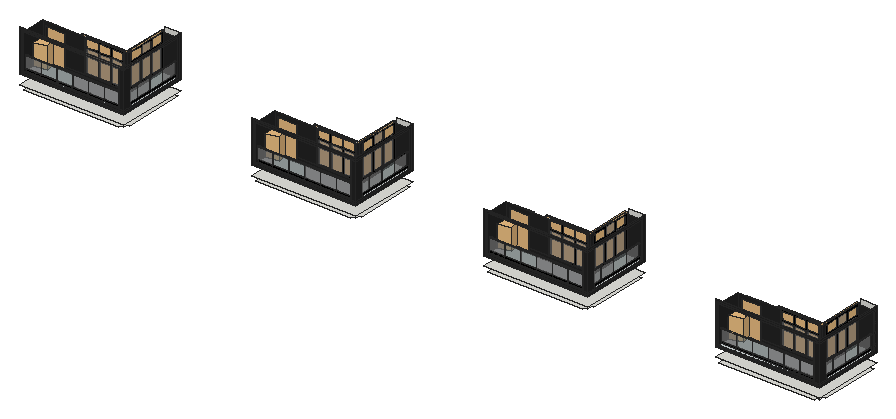
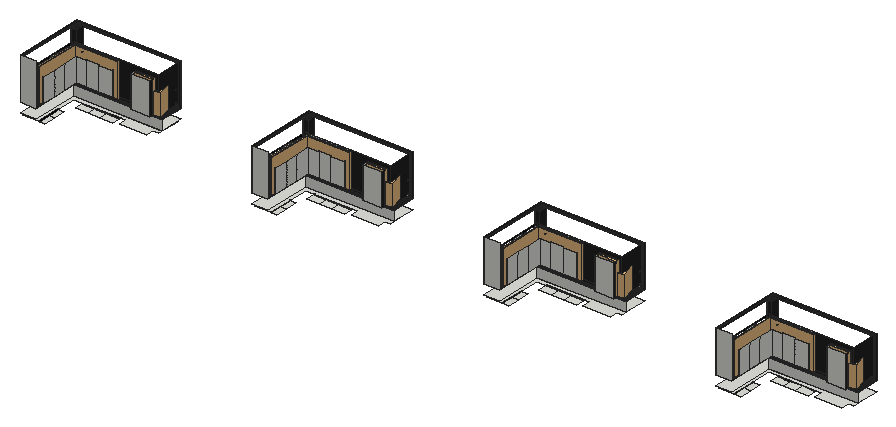
# SketchUp Ruby script. Lengths in inches.
U = 1.inch
M = Sketchup.active_model
def pt(a) = Geom::Point3d.new(a.map { |v| v * U })
def face(e, loops, mat)
  f = e.add_face(loops[0].map { |a| pt(a) })
  loops[1..].each { |l| e.add_face(l.map { |a| pt(a) }).erase! }
  f.material = f.back_material = mat if mat
  f
end
# faces: each face lists its corners as indices into pts; further lists are holes
def faces(e, pts, list, mat = nil) = list.each { |f| face(e, (f[0].is_a?(Array) ? f : [f]).map { |l| l.map { |i| pts[i] } }, mat) }
# xy, xz, yz: faces in a plane at the given z, y or x. An outline is a flat list of corners, or four numbers for a rectangle; further outlines are holes
def ring(l) = l.size == 4 ? [[l[0], l[1]], [l[2], l[1]], [l[2], l[3]], [l[0], l[3]]] : l.each_slice(2).to_a
def flat(e, list, mat, &to3) = list.each { |f| face(e, (f[0].is_a?(Array) ? f : [f]).map { |l| ring(l).map { |u, v| to3.(u, v) } }, mat) }
def xy(e, z, list, mat = nil) = flat(e, list, mat) { |x, y| [x, y, z] }
def xz(e, y, list, mat = nil) = flat(e, list, mat) { |x, z| [x, y, z] }
def yz(e, x, list, mat = nil) = flat(e, list, mat) { |y, z| [x, y, z] }
def lines(e, pts, list) = list.each { |a, b| e.add_line(pt(pts[a]), pt(pts[b])) }
# prism: a flat outline (further loops are holes) pulled along v
def prism(e, loops, v, mat = nil)
  f = face(e, loops, mat); d = Geom::Vector3d.new(v.map { |x| x * U })
  f.pushpull(f.normal.samedirection?(d) ? d.length : -d.length)
end
def box(e, o, s, mat = nil) = prism(e, [[o, [o[0] + s[0], o[1], o[2]], [o[0] + s[0], o[1] + s[1], o[2]], [o[0], o[1] + s[1], o[2]]]], [0, 0, s[2]], mat)
def at(x, y, z, deg = 0) = Geom::Transformation.translation(pt([x, y, z])) * Geom::Transformation.rotation(ORIGIN, Z_AXIS, deg.degrees)
def axes(o, x, y, z) = Geom::Transformation.new([*x, 0, *y, 0, *z, 0, *pt(o).to_a, 1])
def part(name) = M.definitions.add(name)
# library, detail: a bought-in or finely detailed component or shape, given as its bounding box
def library(name, o, s) = part(name).tap { |d| box(d.entities, o, s) }
def detail(e, o, s) = box(e.add_group.entities, o, s)
def put(e, d, t, mat = nil) = e.add_instance(d, t).tap { |i| i.material = mat if mat }
def group(e, t, mat = nil) = e.add_group.tap { |g| g.transformation = t; g.material = mat if mat }.entities
root = M.entities
M.materials.add("Glass Railing Color").color = [198, 198, 198]
M.materials.add("Polycor-Pavers-GEORGIA-MARBLEtm-PEARL-GREY-Tranche-1-4K").color = [207, 214, 215]
M.materials.add("Railing Glass").color = [63, 150, 137]
M.materials["Railing Glass"].alpha = 0.13
M.materials.add("[0136_Charcoal]").color = [35, 35, 35]
M.materials.add("[Color M09]").color = [0, 0, 0]
M.materials.add("[Translucent Glass Gray]").color = [128, 128, 128]
M.materials["[Translucent Glass Gray]"].alpha = 0.5
c1 = library("door by lz",[5.91,-4.92,0],[35.43,6.61,78.74])
c2 = part("Glass Rail Spacer")
box(c2.entities,[-0.5,-0.25,0],[1,0.5,1],"Glass Railing Color")
c3 = part("Group67\#1")
prism(c3.entities,[[[0.54,0,1.27],[0.38,0,1.39],[0.21,0,1.47],[0.01,0,1.5],[-0.18,0,1.48],[-0.37,0,1.41],[-0.52,0,1.29],[-0.64,0,1.13],[-0.72,0,0.96],[-0.75,0,0.76],[-0.73,0,0.57],[-0.66,0,0.38],[-0.54,0,0.23],[-0.38,0,0.11],[-0.21,0,0.03],[-0.01,0,0],[0.18,0,0.02],[0.37,0,0.09],[0.52,0,0.21],[0.64,0,0.37],[0.72,0,0.54],[0.75,0,0.74],[0.73,0,0.93],[0.66,0,1.12]]],[0,242.43,0],"[Color M09]")
c4 = part("Group70\#1")
xy(c4.entities,0,[[-0.5,0,0.5,242.43]],"Glass Railing Color")
xy(c4.entities,4,[[-0.25,0,0.25,242.43]],"Glass Railing Color")
xy(c4.entities,5,[[-0.5,0,-0.25,242.43],[0.25,0,0.5,242.43]],"[Color M09]")
xz(c4.entities,0,[[-0.5,0,0.5,0,0.5,5,0.25,5,0.25,4,-0.25,4,-0.25,5,-0.5,5]],"Glass Railing Color")
xz(c4.entities,242.43,[[-0.5,0,-0.5,5,-0.25,5,-0.25,4,0.25,4,0.25,5,0.5,5,0.5,0]],"Glass Railing Color")
yz(c4.entities,-0.5,[[0,0,242.43,5]],"[Color M09]")
yz(c4.entities,-0.25,[[0,4,242.43,5]],"Glass Railing Color")
yz(c4.entities,0.25,[[0,4,242.43,5]],"[Color M09]")
yz(c4.entities,0.5,[[0,0,242.43,5]],"[Color M09]")
c5 = part("Group71\#1")
box(c5.entities,[-0.1875,0,0],[0.375,39.24,30],"[Translucent Glass Gray]")
c6 = part("Group72\#1")
xy(c6.entities,0,[[-0.1875,0,0.1875,39.24]],"Railing Glass")
xy(c6.entities,30,[[-0.1875,0,0.1875,39.24]],"Railing Glass")
xz(c6.entities,0,[[-0.1875,0,0.1875,30]],"Railing Glass")
xz(c6.entities,39.24,[[-0.1875,0,0.1875,30]],"Railing Glass")
yz(c6.entities,-0.1875,[[0,0,39.24,30]],"Railing Glass")
yz(c6.entities,0.1875,[[0,0,39.24,30]],"[Translucent Glass Gray]")
c7 = part("Group73\#1")
xy(c7.entities,0,[[-0.1875,0,0.1875,39.24]],"Railing Glass")
xy(c7.entities,30,[[-0.1875,0,0.1875,39.24]],"Railing Glass")
xz(c7.entities,0,[[-0.1875,0,0.1875,30]],"Railing Glass")
xz(c7.entities,39.24,[[-0.1875,0,0.1875,30]],"Railing Glass")
yz(c7.entities,-0.1875,[[0,0,39.24,30]],"Railing Glass")
yz(c7.entities,0.1875,[[0,0,39.24,30]],"[Translucent Glass Gray]")
c8 = part("Group74\#1")
box(c8.entities,[-0.1875,0,0],[0.375,39.24,30],"[Translucent Glass Gray]")
c9 = part("Group75\#1")
box(c9.entities,[-0.1875,0,0],[0.375,39.24,30],"[Translucent Glass Gray]")
c10 = part("Group76\#1")
box(c10.entities,[-0.1875,0,0],[0.375,39.24,30],"[Translucent Glass Gray]")
c11 = part("Glass Railing")
put(c11.entities,c2,at(0,0,4))
put(c11.entities,c2,at(40.24,0,4))
put(c11.entities,c2,at(80.48,0,4))
put(c11.entities,c2,at(120.71,0,4))
put(c11.entities,c2,at(160.95,0,4))
put(c11.entities,c2,at(201.19,0,4))
put(c11.entities,c2,at(241.43,0,4))
put(c11.entities,c3,at(-0.5,0,34,-90),"Glass Railing Color")
put(c11.entities,c4,at(-0.5,0,0,-90),"Glass Railing Color")
put(c11.entities,c5,at(0.5,0,4,-90),"Railing Glass")
put(c11.entities,c6,at(40.74,0,4,-90),"Railing Glass")
put(c11.entities,c7,at(80.98,0,4,-90),"Railing Glass")
put(c11.entities,c8,at(121.21,0,4,-90),"Railing Glass")
put(c11.entities,c9,at(161.45,0,4,-90),"Railing Glass")
put(c11.entities,c10,at(201.69,0,4,-90),"Railing Glass")
c12 = part("Group76\#2")
prism(c12.entities,[[[0.54,0,1.27],[0.38,0,1.39],[0.21,0,1.47],[0.01,0,1.5],[-0.18,0,1.48],[-0.37,0,1.41],[-0.52,0,1.29],[-0.64,0,1.13],[-0.72,0,0.96],[-0.75,0,0.76],[-0.73,0,0.57],[-0.66,0,0.38],[-0.54,0,0.23],[-0.38,0,0.11],[-0.21,0,0.03],[-0.01,0,0],[0.18,0,0.02],[0.37,0,0.09],[0.52,0,0.21],[0.64,0,0.37],[0.72,0,0.54],[0.75,0,0.74],[0.73,0,0.93],[0.66,0,1.12]]],[0,161.62,0],"[Color M09]")
c13 = part("Group79\#1")
prism(c13.entities,[[[0.25,0,5],[0.25,0,4],[-0.25,0,4],[-0.25,0,5],[-0.5,0,5],[-0.5,0,0],[0.5,0,0],[0.5,0,5]]],[0,161.62,0],"[Color M09]")
c14 = part("Group80\#1")
box(c14.entities,[-0.1875,0,0],[0.375,39.15,30],"[Translucent Glass Gray]")
c15 = part("Group81\#1")
box(c15.entities,[-0.1875,0,0],[0.375,39.15,30],"[Translucent Glass Gray]")
c16 = part("Group82\#1")
xy(c16.entities,0,[[-0.1875,0,0.1875,39.15]],"Railing Glass")
xy(c16.entities,30,[[-0.1875,0,0.1875,39.15]],"Railing Glass")
xz(c16.entities,0,[[-0.1875,0,0.1875,30]],"Railing Glass")
xz(c16.entities,39.15,[[-0.1875,0,0.1875,30]],"Railing Glass")
yz(c16.entities,-0.1875,[[0,0,39.15,30]],"Railing Glass")
yz(c16.entities,0.1875,[[0,0,39.15,30]],"[Translucent Glass Gray]")
c17 = part("Group83\#1")
box(c17.entities,[-0.1875,0,0],[0.375,39.15,30],"[Translucent Glass Gray]")
c18 = part("Glass Railing\#1")
put(c18.entities,c2,at(0,0,4,90))
put(c18.entities,c2,at(0,40.15,4,90))
put(c18.entities,c2,at(0,80.31,4,90))
put(c18.entities,c2,at(0,120.46,4,90))
put(c18.entities,c2,at(0,160.62,4,90))
put(c18.entities,c12,at(0,-0.5,34),"Glass Railing Color")
put(c18.entities,c13,at(0,-0.5,0),"[Color M09]")
put(c18.entities,c14,at(0,0.5,4),"Railing Glass")
put(c18.entities,c15,at(0,40.65,4),"Railing Glass")
put(c18.entities,c16,at(0,80.81,4),"Railing Glass")
put(c18.entities,c17,at(0,120.96,4),"Railing Glass")
c19 = library("cay+chuoi",[36.12,19.66,0.52],[32.73,35.6,54.38])
c20 = library("curtain",[-132.09,64.9,20.5],[94.35,4.27,84.68])
xy(root,118.1875,[[501.6,560.12,516.04,589.16],[1091.41,560.12,1105.85,589.16],[1681.23,560.12,1695.66,589.16],[2271.04,560.12,2285.48,589.16],[501.6,589.16,516.04,620.2],
  [1091.41,589.16,1105.85,620.2],[1681.23,589.16,1695.66,620.2],[2271.04,589.16,2285.48,620.2]])
xy(root,118.87,[[302.04,449.7,302.04,509.7,315.54,509.7,315.54,530.01,384.73,530.01,384.73,509.7,518.04,509.7,518.04,620.88,557.59,620.88,557.59,468.65,551.21,468.65,551.21,457.2,544.21,457.2,544.21,449.7],[891.85,449.7,891.85,509.7,905.35,509.7,905.35,530.01,974.54,530.01,974.54,509.7,1107.85,509.7,1107.85,620.88,1147.4,620.88,1147.4,468.65,1141.02,468.65,1141.02,457.2,1134.02,457.2,1134.02,449.7],[1481.66,449.7,1481.66,509.7,1495.16,509.7,1495.16,530.01,1564.35,530.01,1564.35,509.7,1697.66,509.7,1697.66,620.88,1737.22,620.88,1737.22,468.65,1730.83,468.65,1730.83,457.2,1723.83,457.2,1723.83,449.7],[2071.48,449.7,2071.48,509.7,2084.98,509.7,2084.98,530.01,2154.16,530.01,2154.16,509.7,2287.48,509.7,2287.48,620.88,2327.03,620.88,2327.03,468.65,2320.65,468.65,2320.65,457.2,2313.65,457.2,2313.65,449.7],[398.04,512.7,430.93,533.7],
  [430.93,512.7,461.15,533.7],[461.15,512.7,494.04,533.7],[987.85,512.7,1020.74,533.7],[1020.74,512.7,1050.96,533.7],[1050.96,512.7,1083.85,533.7],
  [1577.66,512.7,1610.56,533.7],[1610.56,512.7,1640.77,533.7],[1640.77,512.7,1673.66,533.7],[2167.48,512.7,2200.37,533.7],[2200.37,512.7,2230.58,533.7],
  [2230.58,512.7,2263.48,533.7]])
xy(root,118.87,[[398.04,509.7,494.04,512.7],[987.85,509.7,1083.85,512.7],[1577.66,509.7,1673.66,512.7],[2167.48,509.7,2263.48,512.7],[516.04,559.44,518.04,620.88],
  [1105.85,559.44,1107.85,620.88],[1695.66,559.44,1697.66,620.88],[2285.48,559.44,2287.48,620.88]],"[Color M09]")
xy(root,127.6875,[[293.22,449.7,557.59,449.7,557.59,629.7,518.04,629.7,518.04,509.7,293.22,509.7],[883.03,449.7,1147.4,449.7,1147.4,629.7,1107.85,629.7,1107.85,509.7,883.03,509.7],[1472.84,449.7,1737.22,449.7,1737.22,629.7,1697.66,629.7,1697.66,509.7,1472.84,509.7],[2062.65,449.7,2327.03,449.7,2327.03,629.7,2287.48,629.7,2287.48,509.7,2062.65,509.7]])
xy(root,151.6875,[[293.22,449.7,557.59,509.7],[883.03,449.7,1147.4,509.7],[1472.84,449.7,1737.22,509.7],[2062.65,449.7,2327.03,509.7],[518.04,509.7,557.59,629.7],
  [1107.85,509.7,1147.4,629.7],[1697.66,509.7,1737.22,629.7],[2287.48,509.7,2327.03,629.7]],"[0136_Charcoal]")
xy(root,155.16,[[296.69,449.7,557.59,450.7],[886.5,449.7,1147.4,450.7],[1476.32,449.7,1737.22,450.7],[2066.13,449.7,2327.03,450.7],[556.59,450.7,557.59,625.64],
  [1146.4,450.7,1147.4,625.64],[1736.22,450.7,1737.22,625.64],[2326.03,450.7,2327.03,625.64]],"[0136_Charcoal]")
xy(root,156.3,[[297.83,449.7,557.59,450.7],[887.64,449.7,1147.4,450.7],[1477.46,449.7,1737.22,450.7],[2067.27,449.7,2327.03,450.7]],"[0136_Charcoal]")
xy(root,159.6875,[[311.04,509.7,359.04,525.45],[900.85,509.7,948.85,525.45],[1490.66,509.7,1538.66,525.45],[2080.48,509.7,2128.48,525.45]])
xy(root,159.6875,[[302.04,449.7,557.59,449.7,557.59,621.7,518.04,621.7,518.04,509.7,302.04,509.7],[891.85,449.7,1147.4,449.7,1147.4,621.7,1107.85,621.7,1107.85,509.7,891.85,509.7],[1481.66,449.7,1737.22,449.7,1737.22,621.7,1697.66,621.7,1697.66,509.7,1481.66,509.7],[2071.48,449.7,2327.03,449.7,2327.03,621.7,2287.48,621.7,2287.48,509.7,2071.48,509.7]],"Polycor-Pavers-GEORGIA-MARBLEtm-PEARL-GREY-Tranche-1-4K")
xy(root,165.6875,[[410.04,509.7,509.04,511.7],[999.85,509.7,1098.85,511.7],[1589.66,509.7,1688.66,511.7],[2179.48,509.7,2278.48,511.7],[503.73,519.34,515.04,555.96],
  [515.04,519.34,518.04,621.7],[1093.54,519.34,1104.85,555.96],[1104.85,519.34,1107.85,621.7],[1683.35,519.34,1694.66,555.96],[1694.66,519.34,1697.66,621.7],
  [2273.16,519.34,2284.48,555.96],[2284.48,519.34,2287.48,621.7],[503.73,555.96,515.04,588.08],[1093.54,555.96,1104.85,588.08],[1683.35,555.96,1694.66,588.08],
  [2273.16,555.96,2284.48,588.08],[503.73,588.08,515.04,621.7],[1093.54,588.08,1104.85,621.7],[1683.35,588.08,1694.66,621.7],[2273.16,588.08,2284.48,621.7]])
xy(root,166.1875,[[410.54,511.7,445.2,519.01],[445.2,511.7,476.87,519.01],[476.87,511.7,508.54,519.01],[1000.35,511.7,1035.02,519.01],[1035.02,511.7,1066.68,519.01],
  [1066.68,511.7,1098.35,519.01],[1590.16,511.7,1624.83,519.01],[1624.83,511.7,1656.5,519.01],[1656.5,511.7,1688.16,519.01],[2179.98,511.7,2214.64,519.01],
  [2214.64,511.7,2246.31,519.01],[2246.31,511.7,2277.98,519.01]])
xy(root,167.6875,[[445.2,509.7,475.37,511.7],[476.87,509.7,507.04,511.7],[1035.02,509.7,1065.18,511.7],[1066.68,509.7,1096.85,511.7],[1624.83,509.7,1655,511.7],
  [1656.5,509.7,1686.66,511.7],[2214.64,509.7,2244.81,511.7],[2246.31,509.7,2276.48,511.7]])
xy(root,167.6875,[[412.04,509.7,443.7,511.7],[1001.85,509.7,1033.52,511.7],[1591.66,509.7,1623.33,511.7],[2181.48,509.7,2213.14,511.7],[515.04,521.34,518.04,553.96],
  [1104.85,521.34,1107.85,553.96],[1694.66,521.34,1697.66,553.96],[2284.48,521.34,2287.48,553.96],[515.04,555.96,518.04,586.08],[1104.85,555.96,1107.85,586.08],
  [1694.66,555.96,1697.66,586.08],[2284.48,555.96,2287.48,586.08],[515.04,588.08,518.04,619.7],[1104.85,588.08,1107.85,619.7],[1694.66,588.08,1697.66,619.7],
  [2284.48,588.08,2287.48,619.7]],"[Color M09]")
xz(root,449.7,[[293.22,151.6875,557.59,151.6875,557.59,155.16,296.69,155.16,296.69,256.21,557.59,256.21,557.59,259.6875,293.22,259.6875],[883.03,151.6875,1147.4,151.6875,1147.4,155.16,886.5,155.16,886.5,256.21,1147.4,256.21,1147.4,259.6875,883.03,259.6875],[1472.84,151.6875,1737.22,151.6875,1737.22,155.16,1476.32,155.16,1476.32,256.21,1737.22,256.21,1737.22,259.6875,1472.84,259.6875],[2062.65,151.6875,2327.03,151.6875,2327.03,155.16,2066.13,155.16,2066.13,256.21,2327.03,256.21,2327.03,259.6875,2062.65,259.6875],[297.83,156.3,557.59,156.3,557.59,159.6875,302.04,159.6875,302.04,251.6875,557.59,251.6875,557.59,255.07,297.83,255.07],
  [887.64,156.3,1147.4,156.3,1147.4,159.6875,891.85,159.6875,891.85,251.6875,1147.4,251.6875,1147.4,255.07,887.64,255.07],[1477.46,156.3,1737.22,156.3,1737.22,159.6875,1481.66,159.6875,1481.66,251.6875,1737.22,251.6875,1737.22,255.07,1477.46,255.07],[2067.27,156.3,2327.03,156.3,2327.03,159.6875,2071.48,159.6875,2071.48,251.6875,2327.03,251.6875,2327.03,255.07,2067.27,255.07]],"[0136_Charcoal]")
xz(root,450.7,[[296.69,155.16,556.59,155.16,556.59,156.3,297.83,156.3,297.83,255.07,556.59,255.07,556.59,256.21,296.69,256.21],[886.5,155.16,1146.4,155.16,1146.4,156.3,887.64,156.3,887.64,255.07,1146.4,255.07,1146.4,256.21,886.5,256.21],[1476.32,155.16,1736.22,155.16,1736.22,156.3,1477.46,156.3,1477.46,255.07,1736.22,255.07,1736.22,256.21,1476.32,256.21],[2066.13,155.16,2326.03,155.16,2326.03,156.3,2067.27,156.3,2067.27,255.07,2326.03,255.07,2326.03,256.21,2066.13,256.21]],"[0136_Charcoal]")
xz(root,509.7,[[293.22,127.6875,518.04,151.6875],[883.03,127.6875,1107.85,151.6875],[1472.84,127.6875,1697.66,151.6875],[2062.65,127.6875,2287.48,151.6875],[302.04,159.6875,311.04,165.6875],
  [891.85,159.6875,900.85,165.6875],[1481.66,159.6875,1490.66,165.6875],[2071.48,159.6875,2080.48,165.6875]])
xz(root,509.7,[[359.04,159.6875,518.04,165.6875],[948.85,159.6875,1107.85,165.6875],[1538.66,159.6875,1697.66,165.6875],[2128.48,159.6875,2287.48,165.6875],[302.04,165.6875,311.04,165.6875,311.04,240.6,359.04,240.6,359.04,165.6875,410.04,165.6875,410.04,251.6875,302.04,251.6875],
  [509.04,165.6875,518.04,251.6875],[891.85,165.6875,900.85,165.6875,900.85,240.6,948.85,240.6,948.85,165.6875,999.85,165.6875,999.85,251.6875,891.85,251.6875],[1098.85,165.6875,1107.85,251.6875],[1481.66,165.6875,1490.66,165.6875,1490.66,240.6,1538.66,240.6,1538.66,165.6875,1589.66,165.6875,1589.66,251.6875,1481.66,251.6875],[1688.66,165.6875,1697.66,251.6875],
  [2071.48,165.6875,2080.48,165.6875,2080.48,240.6,2128.48,240.6,2128.48,165.6875,2179.48,165.6875,2179.48,251.6875,2071.48,251.6875],[2278.48,165.6875,2287.48,251.6875]],"[0136_Charcoal]")
xz(root,509.7,[[[410.04,165.6875,509.04,251.6875],[412.04,227.74,412.04,249.6875,507.04,249.6875,507.04,227.74,476.87,227.74,476.87,249.6875,475.37,249.6875,475.37,227.74,445.2,227.74,445.2,249.6875,443.7,249.6875,443.7,227.74],[412.04,167.6875,443.7,225.74],[476.87,167.6875,507.04,225.74],[445.2,167.6875,475.37,225.74]],[[999.85,165.6875,1098.85,251.6875],[1001.85,227.74,1001.85,249.6875,1096.85,249.6875,1096.85,227.74,1066.68,227.74,1066.68,249.6875,1065.18,249.6875,1065.18,227.74,1035.02,227.74,1035.02,249.6875,1033.52,249.6875,1033.52,227.74],[1001.85,167.6875,1033.52,225.74],[1066.68,167.6875,1096.85,225.74],[1035.02,167.6875,1065.18,225.74]],[[1589.66,165.6875,1688.66,251.6875],[1591.66,227.74,1591.66,249.6875,1686.66,249.6875,1686.66,227.74,1656.5,227.74,1656.5,249.6875,1655,249.6875,1655,227.74,1624.83,227.74,1624.83,249.6875,1623.33,249.6875,1623.33,227.74],[1591.66,167.6875,1623.33,225.74],[1656.5,167.6875,1686.66,225.74],[1624.83,167.6875,1655,225.74]],[[2179.48,165.6875,2278.48,251.6875],[2181.48,227.74,2181.48,249.6875,2276.48,249.6875,2276.48,227.74,2246.31,227.74,2246.31,249.6875,2244.81,249.6875,2244.81,227.74,2214.64,227.74,2214.64,249.6875,2213.14,249.6875,2213.14,227.74],[2181.48,167.6875,2213.14,225.74],[2246.31,167.6875,2276.48,225.74],[2214.64,167.6875,2244.81,225.74]]],"[Color M09]")
xz(root,510.7,[[476.87,165.6875,509.04,225.74],[1066.68,165.6875,1098.85,225.74],[1656.5,165.6875,1688.66,225.74],[2246.31,165.6875,2278.48,225.74],[412.04,167.6875,443.7,225.74],
  [445.2,167.6875,475.37,225.74],[1001.85,167.6875,1033.52,225.74],[1035.02,167.6875,1065.18,225.74],[1591.66,167.6875,1623.33,225.74],[1624.83,167.6875,1655,225.74],
  [2181.48,167.6875,2213.14,225.74],[2214.64,167.6875,2244.81,225.74]],"[Translucent Glass Gray]")
xz(root,511.7,[[[410.04,165.6875,509.04,251.6875],[410.54,166.1875,508.54,249.6875]],[[999.85,165.6875,1098.85,251.6875],[1000.35,166.1875,1098.35,249.6875]],[[1589.66,165.6875,1688.66,251.6875],[1590.16,166.1875,1688.16,249.6875]],[[2179.48,165.6875,2278.48,251.6875],[2179.98,166.1875,2277.98,249.6875]],[410.54,166.1875,412.04,227.74],
  [412.04,166.1875,443.7,167.6875],[443.7,166.1875,445.2,225.74],[445.2,166.1875,475.37,167.6875],[475.37,166.1875,476.87,227.61],[476.87,166.1875,508.54,167.6875],
  [1000.35,166.1875,1001.85,227.74],[1001.85,166.1875,1033.52,167.6875],[1033.52,166.1875,1035.02,225.74],[1035.02,166.1875,1065.18,167.6875],[1065.18,166.1875,1066.68,227.61],
  [1066.68,166.1875,1098.35,167.6875],[1590.16,166.1875,1591.66,227.74],[1591.66,166.1875,1623.33,167.6875],[1623.33,166.1875,1624.83,225.74],[1624.83,166.1875,1655,167.6875],
  [1655,166.1875,1656.5,227.61],[1656.5,166.1875,1688.16,167.6875],[2179.98,166.1875,2181.48,227.74],[2181.48,166.1875,2213.14,167.6875],[2213.14,166.1875,2214.64,225.74],
  [2214.64,166.1875,2244.81,167.6875],[2244.81,166.1875,2246.31,227.61],[2246.31,166.1875,2277.98,167.6875],[507.04,167.6875,508.54,225.74],[1096.85,167.6875,1098.35,225.74],
  [1686.66,167.6875,1688.16,225.74],[2276.48,167.6875,2277.98,225.74]])
xz(root,519.01,[[410.54,166.1875,445.2,225.74],[445.2,166.1875,476.87,227.61],[476.87,166.1875,508.54,225.74],[1000.35,166.1875,1035.02,225.74],[1035.02,166.1875,1066.68,227.61],
  [1066.68,166.1875,1098.35,225.74],[1590.16,166.1875,1624.83,225.74],[1624.83,166.1875,1656.5,227.61],[1656.5,166.1875,1688.16,225.74],[2179.98,166.1875,2214.64,225.74],
  [2214.64,166.1875,2246.31,227.61],[2246.31,166.1875,2277.98,225.74]])
xz(root,519.34,[[503.73,165.6875,515.04,224.74],[515.04,165.6875,518.04,251.6875],[1093.54,165.6875,1104.85,224.74],[1104.85,165.6875,1107.85,251.6875],[1683.35,165.6875,1694.66,224.74],
  [1694.66,165.6875,1697.66,251.6875],[2273.16,165.6875,2284.48,224.74],[2284.48,165.6875,2287.48,251.6875]])
xz(root,521.34,[[515.04,167.6875,518.04,225.74],[1104.85,167.6875,1107.85,225.74],[1694.66,167.6875,1697.66,225.74],[2284.48,167.6875,2287.48,225.74]],"[Color M09]")
xz(root,525.45,[[311.04,159.6875,359.04,240.6],[900.85,159.6875,948.85,240.6],[1490.66,159.6875,1538.66,240.6],[2080.48,159.6875,2128.48,240.6]])
xz(root,553.96,[[515.04,167.6875,518.04,225.74],[1104.85,167.6875,1107.85,225.74],[1694.66,167.6875,1697.66,225.74],[2284.48,167.6875,2287.48,225.74]],"[Color M09]")
xz(root,555.96,[[515.04,167.6875,518.04,225.74],[1104.85,167.6875,1107.85,225.74],[1694.66,167.6875,1697.66,225.74],[2284.48,167.6875,2287.48,225.74]],"[Color M09]")
xz(root,586.08,[[515.04,167.6875,518.04,225.74],[1104.85,167.6875,1107.85,225.74],[1694.66,167.6875,1697.66,225.74],[2284.48,167.6875,2287.48,225.74]],"[Color M09]")
xz(root,588.08,[[515.04,167.6875,518.04,225.74],[1104.85,167.6875,1107.85,225.74],[1694.66,167.6875,1697.66,225.74],[2284.48,167.6875,2287.48,225.74]],"[Color M09]")
xz(root,619.7,[[515.04,167.6875,518.04,225.74],[1104.85,167.6875,1107.85,225.74],[1694.66,167.6875,1697.66,225.74],[2284.48,167.6875,2287.48,225.74]],"[Color M09]")
xz(root,621.7,[[503.73,165.6875,515.04,224.74],[515.04,165.6875,518.04,251.6875],[1093.54,165.6875,1104.85,224.74],[1104.85,165.6875,1107.85,251.6875],[1683.35,165.6875,1694.66,224.74],
  [1694.66,165.6875,1697.66,251.6875],[2273.16,165.6875,2284.48,224.74],[2284.48,165.6875,2287.48,251.6875]])
xz(root,621.7,[[518.04,159.6875,557.59,251.6875],[1107.85,159.6875,1147.4,251.6875],[1697.66,159.6875,1737.22,251.6875],[2287.48,159.6875,2327.03,251.6875]],"[0136_Charcoal]")
xz(root,624.51,[[556.59,157.14,557.59,255.07],[1146.4,157.14,1147.4,255.07],[1736.22,157.14,1737.22,255.07],[2326.03,157.14,2327.03,255.07]])
xz(root,625.64,[[556.59,155.16,557.59,155.71],[1146.4,155.16,1147.4,155.71],[1736.22,155.16,1737.22,155.71],[2326.03,155.16,2327.03,155.71],[556.59,155.71,557.59,256.21],
  [1146.4,155.71,1147.4,256.21],[1736.22,155.71,1737.22,256.21],[2326.03,155.71,2327.03,256.21]],"[0136_Charcoal]")
xz(root,629.7,[[518.04,151.6875,557.59,259.6875],[1107.85,151.6875,1147.4,259.6875],[1697.66,151.6875,1737.22,259.6875],[2287.48,151.6875,2327.03,259.6875]])
yz(root,296.69,[[449.7,155.16,450.7,256.21]],"[0136_Charcoal]")
yz(root,297.83,[[449.7,156.3,450.7,255.07]],"[0136_Charcoal]")
yz(root,302.04,[[449.7,159.6875,509.7,251.6875]],"[0136_Charcoal]")
yz(root,311.04,[[509.7,159.6875,525.45,240.6]],"[0136_Charcoal]")
yz(root,359.04,[[509.7,159.6875,525.45,240.6]])
yz(root,410.04,[[509.7,165.6875,511.7,251.6875]])
yz(root,410.54,[[511.7,166.1875,519.01,227.74]])
yz(root,412.04,[[509.7,167.6875,511.7,225.74]],"[Color M09]")
yz(root,443.7,[[509.7,167.6875,511.7,225.74]],"[Color M09]")
yz(root,445.2,[[509.7,167.6875,511.7,225.74]],"[Color M09]")
yz(root,475.37,[[509.7,167.6875,511.7,225.74]],"[Color M09]")
yz(root,476.87,[[509.7,167.6875,511.7,225.74]],"[Color M09]")
yz(root,503.73,[[519.34,165.6875,555.96,224.74],[555.96,165.6875,588.08,224.74],[588.08,165.6875,621.7,224.74]])
yz(root,507.04,[[509.7,167.6875,511.7,225.74]],"[Color M09]")
yz(root,508.54,[[511.7,166.1875,519.01,225.74]],"[Color M09]")
yz(root,509.04,[[509.7,165.6875,511.7,251.6875]])
yz(root,515.04,[[519.34,165.6875,519.34,168.6875,521.34,168.6875,521.34,167.6875,552.96,167.6875,552.96,165.6875],[552.96,165.6875,552.96,167.6875,553.96,167.6875,553.96,224.74,555.96,224.74,555.96,165.6875],[555.96,165.6875,585.08,167.6875],[585.08,165.6875,585.08,167.6875,586.08,167.6875,586.08,224.74,588.08,224.74,588.08,165.6875],[588.08,165.6875,618.7,167.6875],
  [618.7,165.6875,618.7,167.6875,619.7,167.6875,619.7,224.74,621.7,224.74,621.7,165.6875]])
yz(root,516.54,[[521.34,167.6875,553.96,225.74],[555.96,167.6875,586.08,225.74],[588.08,167.6875,619.7,225.74],[555.96,225.74,586.08,249.6875]],"[Translucent Glass Gray]")
yz(root,518.04,[[509.7,159.6875,519.34,251.6875],[519.34,159.6875,621.7,165.6875]],"[0136_Charcoal]")
yz(root,518.04,[[[519.34,165.6875,621.7,251.6875],[521.34,167.6875,553.96,225.74],[588.08,167.6875,619.7,225.74],[555.96,167.6875,586.08,225.74],[521.34,227.74,553.96,249.6875],[588.08,227.74,619.7,249.6875],[555.96,227.74,586.08,249.6875]]],"[Color M09]")
yz(root,556.59,[[450.7,155.16,625.64,155.16,625.64,256.21,450.7,256.21,450.7,255.07,624.51,255.07,624.51,157.14,450.7,156.3]],"[0136_Charcoal]")
yz(root,557.59,[[449.7,151.6875,629.7,151.6875,629.7,259.6875,449.7,259.6875,449.7,256.21,625.64,256.21,625.64,155.16,449.7,155.16],[449.7,156.3,450.7,156.3,624.51,157.14,624.51,255.07,449.7,255.07,449.7,251.6875,621.7,251.6875,621.7,159.6875,449.7,159.6875]],"[0136_Charcoal]")
yz(root,886.5,[[449.7,155.16,450.7,256.21]],"[0136_Charcoal]")
yz(root,887.64,[[449.7,156.3,450.7,255.07]],"[0136_Charcoal]")
yz(root,891.85,[[449.7,159.6875,509.7,251.6875]],"[0136_Charcoal]")
yz(root,900.85,[[509.7,159.6875,525.45,240.6]],"[0136_Charcoal]")
yz(root,948.85,[[509.7,159.6875,525.45,240.6]])
yz(root,999.85,[[509.7,165.6875,511.7,251.6875]])
yz(root,1000.35,[[511.7,166.1875,519.01,227.74]])
yz(root,1001.85,[[509.7,167.6875,511.7,225.74]],"[Color M09]")
yz(root,1033.52,[[509.7,167.6875,511.7,225.74]],"[Color M09]")
yz(root,1035.02,[[509.7,167.6875,511.7,225.74]],"[Color M09]")
yz(root,1065.18,[[509.7,167.6875,511.7,225.74]],"[Color M09]")
yz(root,1066.68,[[509.7,167.6875,511.7,225.74]],"[Color M09]")
yz(root,1093.54,[[519.34,165.6875,555.96,224.74],[555.96,165.6875,588.08,224.74],[588.08,165.6875,621.7,224.74]])
yz(root,1096.85,[[509.7,167.6875,511.7,225.74]],"[Color M09]")
yz(root,1098.35,[[511.7,166.1875,519.01,225.74]],"[Color M09]")
yz(root,1098.85,[[509.7,165.6875,511.7,251.6875]])
yz(root,1104.85,[[519.34,165.6875,519.34,168.6875,521.34,168.6875,521.34,167.6875,552.96,167.6875,552.96,165.6875],[552.96,165.6875,552.96,167.6875,553.96,167.6875,553.96,224.74,555.96,224.74,555.96,165.6875],[555.96,165.6875,585.08,167.6875],[585.08,165.6875,585.08,167.6875,586.08,167.6875,586.08,224.74,588.08,224.74,588.08,165.6875],[588.08,165.6875,618.7,167.6875],
  [618.7,165.6875,618.7,167.6875,619.7,167.6875,619.7,224.74,621.7,224.74,621.7,165.6875]])
yz(root,1106.35,[[521.34,167.6875,553.96,225.74],[555.96,167.6875,586.08,225.74],[588.08,167.6875,619.7,225.74],[555.96,225.74,586.08,249.6875]],"[Translucent Glass Gray]")
yz(root,1107.85,[[509.7,159.6875,519.34,251.6875],[519.34,159.6875,621.7,165.6875]],"[0136_Charcoal]")
yz(root,1107.85,[[[519.34,165.6875,621.7,251.6875],[521.34,167.6875,553.96,225.74],[588.08,167.6875,619.7,225.74],[555.96,167.6875,586.08,225.74],[521.34,227.74,553.96,249.6875],[588.08,227.74,619.7,249.6875],[555.96,227.74,586.08,249.6875]]],"[Color M09]")
yz(root,1146.4,[[450.7,155.16,625.64,155.16,625.64,256.21,450.7,256.21,450.7,255.07,624.51,255.07,624.51,157.14,450.7,156.3]],"[0136_Charcoal]")
yz(root,1147.4,[[449.7,151.6875,629.7,151.6875,629.7,259.6875,449.7,259.6875,449.7,256.21,625.64,256.21,625.64,155.16,449.7,155.16],[449.7,156.3,450.7,156.3,624.51,157.14,624.51,255.07,449.7,255.07,449.7,251.6875,621.7,251.6875,621.7,159.6875,449.7,159.6875]],"[0136_Charcoal]")
yz(root,1476.32,[[449.7,155.16,450.7,256.21]],"[0136_Charcoal]")
yz(root,1477.46,[[449.7,156.3,450.7,255.07]],"[0136_Charcoal]")
yz(root,1481.66,[[449.7,159.6875,509.7,251.6875]],"[0136_Charcoal]")
yz(root,1490.66,[[509.7,159.6875,525.45,240.6]],"[0136_Charcoal]")
yz(root,1538.66,[[509.7,159.6875,525.45,240.6]])
yz(root,1589.66,[[509.7,165.6875,511.7,251.6875]])
yz(root,1590.16,[[511.7,166.1875,519.01,227.74]])
yz(root,1591.66,[[509.7,167.6875,511.7,225.74]],"[Color M09]")
yz(root,1623.33,[[509.7,167.6875,511.7,225.74]],"[Color M09]")
yz(root,1624.83,[[509.7,167.6875,511.7,225.74]],"[Color M09]")
yz(root,1655,[[509.7,167.6875,511.7,225.74]],"[Color M09]")
yz(root,1656.5,[[509.7,167.6875,511.7,225.74]],"[Color M09]")
yz(root,1683.35,[[519.34,165.6875,555.96,224.74],[555.96,165.6875,588.08,224.74],[588.08,165.6875,621.7,224.74]])
yz(root,1686.66,[[509.7,167.6875,511.7,225.74]],"[Color M09]")
yz(root,1688.16,[[511.7,166.1875,519.01,225.74]],"[Color M09]")
yz(root,1688.66,[[509.7,165.6875,511.7,251.6875]])
yz(root,1694.66,[[519.34,165.6875,519.34,168.6875,521.34,168.6875,521.34,167.6875,552.96,167.6875,552.96,165.6875],[552.96,165.6875,552.96,167.6875,553.96,167.6875,553.96,224.74,555.96,224.74,555.96,165.6875],[555.96,165.6875,585.08,167.6875],[585.08,165.6875,585.08,167.6875,586.08,167.6875,586.08,224.74,588.08,224.74,588.08,165.6875],[588.08,165.6875,618.7,167.6875],
  [618.7,165.6875,618.7,167.6875,619.7,167.6875,619.7,224.74,621.7,224.74,621.7,165.6875]])
yz(root,1696.16,[[521.34,167.6875,553.96,225.74],[555.96,167.6875,586.08,225.74],[588.08,167.6875,619.7,225.74],[555.96,225.74,586.08,249.6875]],"[Translucent Glass Gray]")
yz(root,1697.66,[[509.7,159.6875,519.34,251.6875],[519.34,159.6875,621.7,165.6875]],"[0136_Charcoal]")
yz(root,1697.66,[[[519.34,165.6875,621.7,251.6875],[521.34,167.6875,553.96,225.74],[588.08,167.6875,619.7,225.74],[555.96,167.6875,586.08,225.74],[521.34,227.74,553.96,249.6875],[588.08,227.74,619.7,249.6875],[555.96,227.74,586.08,249.6875]]],"[Color M09]")
yz(root,1736.22,[[450.7,155.16,625.64,155.16,625.64,256.21,450.7,256.21,450.7,255.07,624.51,255.07,624.51,157.14,450.7,156.3]],"[0136_Charcoal]")
yz(root,1737.22,[[449.7,151.6875,629.7,151.6875,629.7,259.6875,449.7,259.6875,449.7,256.21,625.64,256.21,625.64,155.16,449.7,155.16],[449.7,156.3,450.7,156.3,624.51,157.14,624.51,255.07,449.7,255.07,449.7,251.6875,621.7,251.6875,621.7,159.6875,449.7,159.6875]],"[0136_Charcoal]")
yz(root,2066.13,[[449.7,155.16,450.7,256.21]],"[0136_Charcoal]")
yz(root,2067.27,[[449.7,156.3,450.7,255.07]],"[0136_Charcoal]")
yz(root,2071.48,[[449.7,159.6875,509.7,251.6875]],"[0136_Charcoal]")
yz(root,2080.48,[[509.7,159.6875,525.45,240.6]],"[0136_Charcoal]")
yz(root,2128.48,[[509.7,159.6875,525.45,240.6]])
yz(root,2179.48,[[509.7,165.6875,511.7,251.6875]])
yz(root,2179.98,[[511.7,166.1875,519.01,227.74]])
yz(root,2181.48,[[509.7,167.6875,511.7,225.74]],"[Color M09]")
yz(root,2213.14,[[509.7,167.6875,511.7,225.74]],"[Color M09]")
yz(root,2214.64,[[509.7,167.6875,511.7,225.74]],"[Color M09]")
yz(root,2244.81,[[509.7,167.6875,511.7,225.74]],"[Color M09]")
yz(root,2246.31,[[509.7,167.6875,511.7,225.74]],"[Color M09]")
yz(root,2273.16,[[519.34,165.6875,555.96,224.74],[555.96,165.6875,588.08,224.74],[588.08,165.6875,621.7,224.74]])
yz(root,2276.48,[[509.7,167.6875,511.7,225.74]],"[Color M09]")
yz(root,2277.98,[[511.7,166.1875,519.01,225.74]],"[Color M09]")
yz(root,2278.48,[[509.7,165.6875,511.7,251.6875]])
yz(root,2284.48,[[519.34,165.6875,519.34,168.6875,521.34,168.6875,521.34,167.6875,552.96,167.6875,552.96,165.6875],[552.96,165.6875,552.96,167.6875,553.96,167.6875,553.96,224.74,555.96,224.74,555.96,165.6875],[555.96,165.6875,585.08,167.6875],[585.08,165.6875,585.08,167.6875,586.08,167.6875,586.08,224.74,588.08,224.74,588.08,165.6875],[588.08,165.6875,618.7,167.6875],
  [618.7,165.6875,618.7,167.6875,619.7,167.6875,619.7,224.74,621.7,224.74,621.7,165.6875]])
yz(root,2285.98,[[521.34,167.6875,553.96,225.74],[555.96,167.6875,586.08,225.74],[588.08,167.6875,619.7,225.74],[555.96,225.74,586.08,249.6875]],"[Translucent Glass Gray]")
yz(root,2287.48,[[509.7,159.6875,519.34,251.6875],[519.34,159.6875,621.7,165.6875]],"[0136_Charcoal]")
yz(root,2287.48,[[[519.34,165.6875,621.7,251.6875],[521.34,167.6875,553.96,225.74],[588.08,167.6875,619.7,225.74],[555.96,167.6875,586.08,225.74],[521.34,227.74,553.96,249.6875],[588.08,227.74,619.7,249.6875],[555.96,227.74,586.08,249.6875]]],"[Color M09]")
yz(root,2326.03,[[450.7,155.16,625.64,155.16,625.64,256.21,450.7,256.21,450.7,255.07,624.51,255.07,624.51,157.14,450.7,156.3]],"[0136_Charcoal]")
yz(root,2327.03,[[449.7,151.6875,629.7,151.6875,629.7,259.6875,449.7,259.6875,449.7,256.21,625.64,256.21,625.64,155.16,449.7,155.16],[449.7,156.3,450.7,156.3,624.51,157.14,624.51,255.07,449.7,255.07,449.7,251.6875,621.7,251.6875,621.7,159.6875,449.7,159.6875]],"[0136_Charcoal]")
p = [[557.59,624.51,157.14],[557.59,450.7,156.3],[556.59,450.7,156.3],[556.59,624.51,157.14],[1147.4,624.51,157.14],[1147.4,450.7,156.3],
  [1146.4,450.7,156.3],[1146.4,624.51,157.14],[1737.22,624.51,157.14],[1737.22,450.7,156.3],[1736.22,450.7,156.3],[1736.22,624.51,157.14],
  [2327.03,624.51,157.14],[2327.03,450.7,156.3],[2326.03,450.7,156.3],[2326.03,624.51,157.14]]
faces(root,p,[[0,1,2,3],[4,5,6,7],[8,9,10,11],[12,13,14,15]])
put(root,c1,axes([303.03,515.51,159.6875],[1.35467,0,0],[0,1,0],[0,0,1.02753]))
put(root,c1,axes([892.84,515.51,159.6875],[1.35467,0,0],[0,1,0],[0,0,1.02753]))
put(root,c1,axes([1482.65,515.51,159.6875],[1.35467,0,0],[0,1,0],[0,0,1.02753]))
put(root,c1,axes([2072.47,515.51,159.6875],[1.35467,0,0],[0,1,0],[0,0,1.02753]))
g1 = group(root,at(538.84,447.76,159.6875),"[0136_Charcoal]")
box(g1,[4.625,1.9375,0],[14.125,18.94,92])
put(root,c11,at(302.04,456.08,159.6875))
put(root,c18,at(550.53,461.08,159.6875))
g2 = group(root,at(1128.65,447.76,159.6875),"[0136_Charcoal]")
box(g2,[4.625,1.9375,0],[14.125,18.94,92])
put(root,c11,at(891.85,456.08,159.6875))
put(root,c18,at(1140.34,461.08,159.6875))
g3 = group(root,at(1718.47,447.76,159.6875),"[0136_Charcoal]")
box(g3,[4.625,1.9375,0],[14.125,18.94,92])
put(root,c11,at(1481.66,456.08,159.6875))
put(root,c18,at(1730.15,461.08,159.6875))
g4 = group(root,at(2308.28,447.76,159.6875),"[0136_Charcoal]")
box(g4,[4.625,1.9375,0],[14.125,18.94,92])
put(root,c11,at(2071.48,456.08,159.6875))
put(root,c18,at(2319.97,461.08,159.6875))
put(root,c19,at(272.97,449.07,159.875,15))
put(root,c19,at(862.79,449.07,159.875,15))
put(root,c19,at(1452.6,449.07,159.875,15))
put(root,c19,at(2042.41,449.07,159.875,15))
put(root,c20,axes([577.375,674.18,144.39],[0,1.18,0],[-1,0,0],[0,0,1]))
put(root,c20,axes([1167.1875,674.18,144.39],[0,1.18,0],[-1,0,0],[0,0,1]))
put(root,c20,axes([1757,674.18,144.39],[0,1.18,0],[-1,0,0],[0,0,1]))
put(root,c20,axes([2346.8125,674.18,144.39],[0,1.18,0],[-1,0,0],[0,0,1]))
put(root,c20,axes([553.9,449.7,145.6],[1.18,0,0],[0,1,0],[0,0,1]))
put(root,c20,axes([1143.72,449.7,145.6],[1.18,0,0],[0,1,0],[0,0,1]))
put(root,c20,axes([1733.53,449.7,145.6],[1.18,0,0],[0,1,0],[0,0,1]))
put(root,c20,axes([2323.34,449.7,145.6],[1.18,0,0],[0,1,0],[0,0,1]))
